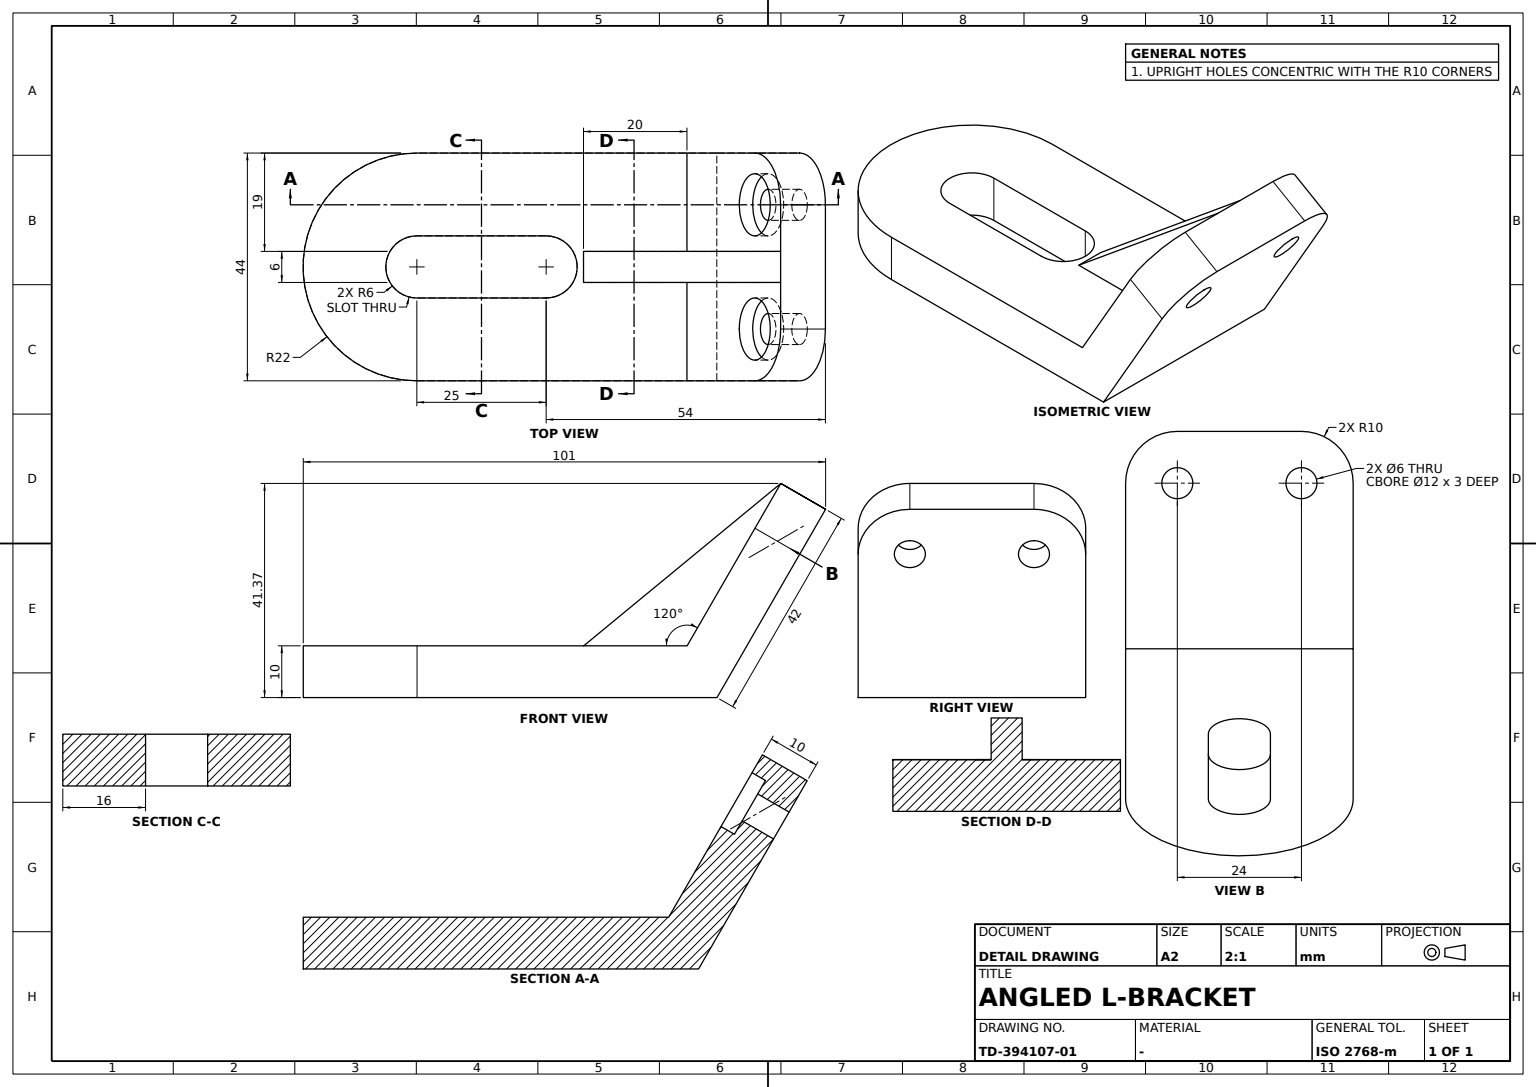
ISO-10303-21;
HEADER;
FILE_DESCRIPTION((''),'2;1');
FILE_NAME('','',(''),(''),'','','');
FILE_SCHEMA(('AUTOMOTIVE_DESIGN'));
ENDSEC;
DATA;
#1=APPLICATION_CONTEXT('');
#2=PRODUCT_CONTEXT('',#1,'mechanical');
#3=PRODUCT('','','',(#2));
#4=PRODUCT_DEFINITION_FORMATION('','',#3);
#5=PRODUCT_DEFINITION_CONTEXT('',#1,'design');
#6=PRODUCT_DEFINITION('','',#4,#5);
#7=PRODUCT_DEFINITION_SHAPE('','',#6);
#8=(LENGTH_UNIT()NAMED_UNIT(*)SI_UNIT(.MILLI.,.METRE.));
#9=(NAMED_UNIT(*)PLANE_ANGLE_UNIT()SI_UNIT($,.RADIAN.));
#10=(NAMED_UNIT(*)SI_UNIT($,.STERADIAN.)SOLID_ANGLE_UNIT());
#11=UNCERTAINTY_MEASURE_WITH_UNIT(LENGTH_MEASURE(0.005),#8,'distance_accuracy_value','');
#12=(GEOMETRIC_REPRESENTATION_CONTEXT(3)GLOBAL_UNCERTAINTY_ASSIGNED_CONTEXT((#11))GLOBAL_UNIT_ASSIGNED_CONTEXT((#8,#9,#10))REPRESENTATION_CONTEXT('',''));
#13=CARTESIAN_POINT('',(33.,6.,0.));
#14=VERTEX_POINT('',#13);
#15=CARTESIAN_POINT('',(33.,6.,10.));
#16=VERTEX_POINT('',#15);
#17=CARTESIAN_POINT('',(33.,6.,5.));
#18=DIRECTION('',(0.,0.,1.));
#19=VECTOR('',#18,1000.);
#20=LINE('',#17,#19);
#21=EDGE_CURVE('',#14,#16,#20,.T.);
#22=ORIENTED_EDGE('',*,*,#21,.T.);
#23=CARTESIAN_POINT('',(33.,-6.,10.));
#24=VERTEX_POINT('',#23);
#25=CARTESIAN_POINT('',(33.,0.,10.));
#26=DIRECTION('',(1.,0.,0.));
#27=AXIS2_PLACEMENT_3D('',#25,#18,#26);
#28=CIRCLE('',#27,6.);
#29=EDGE_CURVE('',#16,#24,#28,.T.);
#30=ORIENTED_EDGE('',*,*,#29,.T.);
#31=CARTESIAN_POINT('',(33.,-6.,0.));
#32=VERTEX_POINT('',#31);
#33=CARTESIAN_POINT('',(33.,-6.,5.));
#34=LINE('',#33,#19);
#35=EDGE_CURVE('',#32,#24,#34,.T.);
#36=ORIENTED_EDGE('',*,*,#35,.F.);
#37=CARTESIAN_POINT('',(33.,0.,0.));
#38=AXIS2_PLACEMENT_3D('',#37,#18,#26);
#39=CIRCLE('',#38,6.);
#40=EDGE_CURVE('',#14,#32,#39,.T.);
#41=ORIENTED_EDGE('',*,*,#40,.F.);
#42=EDGE_LOOP('',(#22,#30,#36,#41));
#43=FACE_BOUND('',#42,.T.);
#44=CARTESIAN_POINT('',(33.,0.,5.));
#45=AXIS2_PLACEMENT_3D('',#44,#18,#26);
#46=CYLINDRICAL_SURFACE('',#45,6.);
#47=ADVANCED_FACE('',(#43),#46,.F.);
#48=CARTESIAN_POINT('',(-4.339746,12.,27.51666));
#49=VERTEX_POINT('',#48);
#50=CARTESIAN_POINT('',(-7.339746,12.,32.712813));
#51=DIRECTION('',(0.866025404,0.,0.5));
#52=DIRECTION('',(0.5,0.,-0.866025404));
#53=AXIS2_PLACEMENT_3D('',#50,#51,#52);
#54=CIRCLE('',#53,6.);
#55=EDGE_CURVE('',#49,#49,#54,.T.);
#56=ORIENTED_EDGE('',*,*,#55,.F.);
#57=EDGE_LOOP('',(#56));
#58=FACE_BOUND('',#57,.T.);
#59=CARTESIAN_POINT('',(5.773503,3.,10.));
#60=VERTEX_POINT('',#59);
#61=CARTESIAN_POINT('',(5.773503,22.,10.));
#62=VERTEX_POINT('',#61);
#63=CARTESIAN_POINT('',(5.773503,0.,10.));
#64=DIRECTION('',(0.,1.,0.));
#65=VECTOR('',#64,1000.);
#66=LINE('',#63,#65);
#67=EDGE_CURVE('',#60,#62,#66,.T.);
#68=ORIENTED_EDGE('',*,*,#67,.T.);
#69=CARTESIAN_POINT('',(-7.339746,22.,32.712813));
#70=VERTEX_POINT('',#69);
#71=CARTESIAN_POINT('',(23.160254,22.,-20.114737));
#72=VECTOR('',#52,1000.);
#73=LINE('',#71,#72);
#74=EDGE_CURVE('',#70,#62,#73,.T.);
#75=ORIENTED_EDGE('',*,*,#74,.F.);
#76=CARTESIAN_POINT('',(-12.339746,12.,41.373067));
#77=VERTEX_POINT('',#76);
#78=CIRCLE('',#53,10.);
#79=EDGE_CURVE('',#70,#77,#78,.T.);
#80=ORIENTED_EDGE('',*,*,#79,.T.);
#81=CARTESIAN_POINT('',(-12.339746,3.,41.373067));
#82=VERTEX_POINT('',#81);
#83=CARTESIAN_POINT('',(-12.339746,-22.,41.373067));
#84=LINE('',#83,#65);
#85=EDGE_CURVE('',#82,#77,#84,.T.);
#86=ORIENTED_EDGE('',*,*,#85,.F.);
#87=CARTESIAN_POINT('',(8.660254,3.,5.));
#88=LINE('',#87,#72);
#89=EDGE_CURVE('',#82,#60,#88,.T.);
#90=ORIENTED_EDGE('',*,*,#89,.T.);
#91=EDGE_LOOP('',(#68,#75,#80,#86,#90));
#92=FACE_BOUND('',#91,.T.);
#93=AXIS2_PLACEMENT_3D('',#83,#51,#52);
#94=PLANE('',#93);
#95=ADVANCED_FACE('',(#58,#92),#94,.T.);
#96=CARTESIAN_POINT('',(58.,-6.,0.));
#97=VERTEX_POINT('',#96);
#98=CARTESIAN_POINT('',(58.,6.,0.));
#99=VERTEX_POINT('',#98);
#100=CARTESIAN_POINT('',(58.,0.,0.));
#101=AXIS2_PLACEMENT_3D('',#100,#18,#26);
#102=CIRCLE('',#101,6.);
#103=EDGE_CURVE('',#97,#99,#102,.T.);
#104=ORIENTED_EDGE('',*,*,#103,.F.);
#105=CARTESIAN_POINT('',(58.,-6.,10.));
#106=VERTEX_POINT('',#105);
#107=CARTESIAN_POINT('',(58.,-6.,5.));
#108=LINE('',#107,#19);
#109=EDGE_CURVE('',#97,#106,#108,.T.);
#110=ORIENTED_EDGE('',*,*,#109,.T.);
#111=CARTESIAN_POINT('',(58.,6.,10.));
#112=VERTEX_POINT('',#111);
#113=CARTESIAN_POINT('',(58.,0.,10.));
#114=AXIS2_PLACEMENT_3D('',#113,#18,#26);
#115=CIRCLE('',#114,6.);
#116=EDGE_CURVE('',#106,#112,#115,.T.);
#117=ORIENTED_EDGE('',*,*,#116,.T.);
#118=CARTESIAN_POINT('',(58.,6.,5.));
#119=LINE('',#118,#19);
#120=EDGE_CURVE('',#99,#112,#119,.T.);
#121=ORIENTED_EDGE('',*,*,#120,.F.);
#122=EDGE_LOOP('',(#104,#110,#117,#121));
#123=FACE_BOUND('',#122,.T.);
#124=CARTESIAN_POINT('',(58.,0.,5.));
#125=AXIS2_PLACEMENT_3D('',#124,#18,#26);
#126=CYLINDRICAL_SURFACE('',#125,6.);
#127=ADVANCED_FACE('',(#123),#126,.F.);
#128=CARTESIAN_POINT('',(-8.437822,-12.,28.614737));
#129=VERTEX_POINT('',#128);
#130=CARTESIAN_POINT('',(-9.937822,-12.,31.212813));
#131=AXIS2_PLACEMENT_3D('',#130,#51,#52);
#132=CIRCLE('',#131,3.);
#133=EDGE_CURVE('',#129,#129,#132,.T.);
#134=ORIENTED_EDGE('',*,*,#133,.F.);
#135=EDGE_LOOP('',(#134));
#136=FACE_BOUND('',#135,.T.);
#137=CARTESIAN_POINT('',(-6.937822,-12.,26.01666));
#138=VERTEX_POINT('',#137);
#139=CIRCLE('',#131,6.);
#140=EDGE_CURVE('',#138,#138,#139,.T.);
#141=ORIENTED_EDGE('',*,*,#140,.T.);
#142=EDGE_LOOP('',(#141));
#143=FACE_BOUND('',#142,.T.);
#144=CARTESIAN_POINT('',(6.062178,0.,3.5));
#145=AXIS2_PLACEMENT_3D('',#144,#51,#64);
#146=PLANE('',#145);
#147=ADVANCED_FACE('',(#136,#143),#146,.T.);
#148=CARTESIAN_POINT('',(-7.339746,-22.,32.712813));
#149=VERTEX_POINT('',#148);
#150=CARTESIAN_POINT('',(5.773503,-22.,10.));
#151=VERTEX_POINT('',#150);
#152=LINE('',#83,#72);
#153=EDGE_CURVE('',#149,#151,#152,.T.);
#154=ORIENTED_EDGE('',*,*,#153,.F.);
#155=CARTESIAN_POINT('',(-16.,-22.,27.712813));
#156=VERTEX_POINT('',#155);
#157=CARTESIAN_POINT('',(-7.403848,-22.,32.675804));
#158=VECTOR('',#51,1000.);
#159=LINE('',#157,#158);
#160=EDGE_CURVE('',#156,#149,#159,.T.);
#161=ORIENTED_EDGE('',*,*,#160,.F.);
#162=CARTESIAN_POINT('',(0.,-22.,0.));
#163=VERTEX_POINT('',#162);
#164=DIRECTION('',(-0.5,0.,0.866025404));
#165=VECTOR('',#164,1000.);
#166=LINE('',#162,#165);
#167=EDGE_CURVE('',#163,#156,#166,.T.);
#168=ORIENTED_EDGE('',*,*,#167,.F.);
#169=CARTESIAN_POINT('',(58.,-22.,0.));
#170=VERTEX_POINT('',#169);
#171=VECTOR('',#26,1000.);
#172=LINE('',#162,#171);
#173=EDGE_CURVE('',#163,#170,#172,.T.);
#174=ORIENTED_EDGE('',*,*,#173,.T.);
#175=CARTESIAN_POINT('',(58.,-22.,10.));
#176=VERTEX_POINT('',#175);
#177=CARTESIAN_POINT('',(58.,-22.,5.));
#178=LINE('',#177,#19);
#179=EDGE_CURVE('',#170,#176,#178,.T.);
#180=ORIENTED_EDGE('',*,*,#179,.T.);
#181=CARTESIAN_POINT('',(0.,-22.,10.));
#182=LINE('',#181,#171);
#183=EDGE_CURVE('',#151,#176,#182,.T.);
#184=ORIENTED_EDGE('',*,*,#183,.F.);
#185=EDGE_LOOP('',(#154,#161,#168,#174,#180,#184));
#186=FACE_BOUND('',#185,.T.);
#187=DIRECTION('',(0.,-1.,0.));
#188=AXIS2_PLACEMENT_3D('',#162,#187,#26);
#189=PLANE('',#188);
#190=ADVANCED_FACE('',(#186),#189,.T.);
#191=CARTESIAN_POINT('',(-12.339746,-12.,41.373067));
#192=VERTEX_POINT('',#191);
#193=CARTESIAN_POINT('',(-12.339746,-3.,41.373067));
#194=VERTEX_POINT('',#193);
#195=EDGE_CURVE('',#192,#194,#84,.T.);
#196=ORIENTED_EDGE('',*,*,#195,.F.);
#197=CARTESIAN_POINT('',(-7.339746,-12.,32.712813));
#198=AXIS2_PLACEMENT_3D('',#197,#51,#52);
#199=CIRCLE('',#198,10.);
#200=EDGE_CURVE('',#192,#149,#199,.T.);
#201=ORIENTED_EDGE('',*,*,#200,.T.);
#202=ORIENTED_EDGE('',*,*,#153,.T.);
#203=CARTESIAN_POINT('',(5.773503,-3.,10.));
#204=VERTEX_POINT('',#203);
#205=EDGE_CURVE('',#151,#204,#66,.T.);
#206=ORIENTED_EDGE('',*,*,#205,.T.);
#207=CARTESIAN_POINT('',(8.660254,-3.,5.));
#208=LINE('',#207,#72);
#209=EDGE_CURVE('',#194,#204,#208,.T.);
#210=ORIENTED_EDGE('',*,*,#209,.F.);
#211=EDGE_LOOP('',(#196,#201,#202,#206,#210));
#212=FACE_BOUND('',#211,.T.);
#213=CARTESIAN_POINT('',(-4.339746,-12.,27.51666));
#214=VERTEX_POINT('',#213);
#215=CIRCLE('',#198,6.);
#216=EDGE_CURVE('',#214,#214,#215,.T.);
#217=ORIENTED_EDGE('',*,*,#216,.F.);
#218=EDGE_LOOP('',(#217));
#219=FACE_BOUND('',#218,.T.);
#220=ADVANCED_FACE('',(#212,#219),#94,.T.);
#221=CARTESIAN_POINT('',(-17.5,12.,30.310889));
#222=VERTEX_POINT('',#221);
#223=CARTESIAN_POINT('',(-16.,12.,27.712813));
#224=DIRECTION('',(-0.866025404,0.,-0.5));
#225=AXIS2_PLACEMENT_3D('',#223,#224,#164);
#226=CIRCLE('',#225,3.);
#227=EDGE_CURVE('',#222,#222,#226,.T.);
#228=ORIENTED_EDGE('',*,*,#227,.F.);
#229=EDGE_LOOP('',(#228));
#230=FACE_BOUND('',#229,.T.);
#231=CARTESIAN_POINT('',(-17.5,-12.,30.310889));
#232=VERTEX_POINT('',#231);
#233=CARTESIAN_POINT('',(-16.,-12.,27.712813));
#234=AXIS2_PLACEMENT_3D('',#233,#224,#164);
#235=CIRCLE('',#234,3.);
#236=EDGE_CURVE('',#232,#232,#235,.T.);
#237=ORIENTED_EDGE('',*,*,#236,.F.);
#238=EDGE_LOOP('',(#237));
#239=FACE_BOUND('',#238,.T.);
#240=CARTESIAN_POINT('',(0.,22.,0.));
#241=VERTEX_POINT('',#240);
#242=CARTESIAN_POINT('',(0.,0.,0.));
#243=VECTOR('',#187,1000.);
#244=LINE('',#242,#243);
#245=EDGE_CURVE('',#241,#163,#244,.T.);
#246=ORIENTED_EDGE('',*,*,#245,.T.);
#247=ORIENTED_EDGE('',*,*,#167,.T.);
#248=CARTESIAN_POINT('',(-21.,-12.,36.373067));
#249=VERTEX_POINT('',#248);
#250=CIRCLE('',#234,10.);
#251=EDGE_CURVE('',#156,#249,#250,.T.);
#252=ORIENTED_EDGE('',*,*,#251,.T.);
#253=CARTESIAN_POINT('',(-21.,12.,36.373067));
#254=VERTEX_POINT('',#253);
#255=CARTESIAN_POINT('',(-21.,-22.,36.373067));
#256=LINE('',#255,#65);
#257=EDGE_CURVE('',#249,#254,#256,.T.);
#258=ORIENTED_EDGE('',*,*,#257,.T.);
#259=CARTESIAN_POINT('',(-16.,22.,27.712813));
#260=VERTEX_POINT('',#259);
#261=CIRCLE('',#225,10.);
#262=EDGE_CURVE('',#254,#260,#261,.T.);
#263=ORIENTED_EDGE('',*,*,#262,.T.);
#264=CARTESIAN_POINT('',(14.5,22.,-25.114737));
#265=LINE('',#264,#165);
#266=EDGE_CURVE('',#241,#260,#265,.T.);
#267=ORIENTED_EDGE('',*,*,#266,.F.);
#268=EDGE_LOOP('',(#246,#247,#252,#258,#263,#267));
#269=FACE_BOUND('',#268,.T.);
#270=AXIS2_PLACEMENT_3D('',#162,#224,#164);
#271=PLANE('',#270);
#272=ADVANCED_FACE('',(#230,#239,#269),#271,.T.);
#273=ORIENTED_EDGE('',*,*,#251,.F.);
#274=ORIENTED_EDGE('',*,*,#160,.T.);
#275=ORIENTED_EDGE('',*,*,#200,.F.);
#276=CARTESIAN_POINT('',(-12.403848,-12.,41.336058));
#277=LINE('',#276,#158);
#278=EDGE_CURVE('',#249,#192,#277,.T.);
#279=ORIENTED_EDGE('',*,*,#278,.F.);
#280=EDGE_LOOP('',(#273,#274,#275,#279));
#281=FACE_BOUND('',#280,.T.);
#282=CARTESIAN_POINT('',(-7.403848,-12.,32.675804));
#283=AXIS2_PLACEMENT_3D('',#282,#51,#164);
#284=CYLINDRICAL_SURFACE('',#283,10.);
#285=ADVANCED_FACE('',(#281),#284,.T.);
#286=ORIENTED_EDGE('',*,*,#29,.F.);
#287=CARTESIAN_POINT('',(0.,6.,10.));
#288=LINE('',#287,#171);
#289=EDGE_CURVE('',#16,#112,#288,.T.);
#290=ORIENTED_EDGE('',*,*,#289,.T.);
#291=ORIENTED_EDGE('',*,*,#116,.F.);
#292=CARTESIAN_POINT('',(0.,-6.,10.));
#293=LINE('',#292,#171);
#294=EDGE_CURVE('',#24,#106,#293,.T.);
#295=ORIENTED_EDGE('',*,*,#294,.F.);
#296=EDGE_LOOP('',(#286,#290,#291,#295));
#297=FACE_BOUND('',#296,.T.);
#298=CARTESIAN_POINT('',(58.,22.,10.));
#299=VERTEX_POINT('',#298);
#300=CARTESIAN_POINT('',(0.,22.,10.));
#301=DIRECTION('',(-1.,0.,0.));
#302=VECTOR('',#301,1000.);
#303=LINE('',#300,#302);
#304=EDGE_CURVE('',#299,#62,#303,.T.);
#305=ORIENTED_EDGE('',*,*,#304,.T.);
#306=ORIENTED_EDGE('',*,*,#67,.F.);
#307=CARTESIAN_POINT('',(25.773503,3.,10.));
#308=VERTEX_POINT('',#307);
#309=CARTESIAN_POINT('',(0.,3.,10.));
#310=LINE('',#309,#171);
#311=EDGE_CURVE('',#60,#308,#310,.T.);
#312=ORIENTED_EDGE('',*,*,#311,.T.);
#313=CARTESIAN_POINT('',(25.773503,-3.,10.));
#314=VERTEX_POINT('',#313);
#315=CARTESIAN_POINT('',(25.773503,0.,10.));
#316=LINE('',#315,#65);
#317=EDGE_CURVE('',#314,#308,#316,.T.);
#318=ORIENTED_EDGE('',*,*,#317,.F.);
#319=CARTESIAN_POINT('',(0.,-3.,10.));
#320=LINE('',#319,#171);
#321=EDGE_CURVE('',#204,#314,#320,.T.);
#322=ORIENTED_EDGE('',*,*,#321,.F.);
#323=ORIENTED_EDGE('',*,*,#205,.F.);
#324=ORIENTED_EDGE('',*,*,#183,.T.);
#325=CIRCLE('',#114,22.);
#326=EDGE_CURVE('',#176,#299,#325,.T.);
#327=ORIENTED_EDGE('',*,*,#326,.T.);
#328=EDGE_LOOP('',(#305,#306,#312,#318,#322,#323,#324,#327));
#329=FACE_BOUND('',#328,.T.);
#330=CARTESIAN_POINT('',(0.,0.,10.));
#331=AXIS2_PLACEMENT_3D('',#330,#18,#26);
#332=PLANE('',#331);
#333=ADVANCED_FACE('',(#297,#329),#332,.T.);
#334=ORIENTED_EDGE('',*,*,#278,.T.);
#335=ORIENTED_EDGE('',*,*,#195,.T.);
#336=LINE('',#83,#243);
#337=EDGE_CURVE('',#82,#194,#336,.T.);
#338=ORIENTED_EDGE('',*,*,#337,.F.);
#339=ORIENTED_EDGE('',*,*,#85,.T.);
#340=CARTESIAN_POINT('',(-12.403848,12.,41.336058));
#341=LINE('',#340,#158);
#342=EDGE_CURVE('',#254,#77,#341,.T.);
#343=ORIENTED_EDGE('',*,*,#342,.F.);
#344=ORIENTED_EDGE('',*,*,#257,.F.);
#345=EDGE_LOOP('',(#334,#335,#338,#339,#343,#344));
#346=FACE_BOUND('',#345,.T.);
#347=AXIS2_PLACEMENT_3D('',#255,#164,#51);
#348=PLANE('',#347);
#349=ADVANCED_FACE('',(#346),#348,.T.);
#350=CARTESIAN_POINT('',(-6.937822,12.,26.01666));
#351=VERTEX_POINT('',#350);
#352=CARTESIAN_POINT('',(-9.937822,12.,31.212813));
#353=AXIS2_PLACEMENT_3D('',#352,#51,#52);
#354=CIRCLE('',#353,6.);
#355=EDGE_CURVE('',#351,#351,#354,.T.);
#356=ORIENTED_EDGE('',*,*,#355,.T.);
#357=EDGE_LOOP('',(#356));
#358=FACE_BOUND('',#357,.T.);
#359=CARTESIAN_POINT('',(-8.437822,12.,28.614737));
#360=VERTEX_POINT('',#359);
#361=CIRCLE('',#353,3.);
#362=EDGE_CURVE('',#360,#360,#361,.T.);
#363=ORIENTED_EDGE('',*,*,#362,.F.);
#364=EDGE_LOOP('',(#363));
#365=FACE_BOUND('',#364,.T.);
#366=ADVANCED_FACE('',(#358,#365),#146,.T.);
#367=ORIENTED_EDGE('',*,*,#109,.F.);
#368=CARTESIAN_POINT('',(0.,-6.,0.));
#369=LINE('',#368,#171);
#370=EDGE_CURVE('',#32,#97,#369,.T.);
#371=ORIENTED_EDGE('',*,*,#370,.F.);
#372=ORIENTED_EDGE('',*,*,#35,.T.);
#373=ORIENTED_EDGE('',*,*,#294,.T.);
#374=EDGE_LOOP('',(#367,#371,#372,#373));
#375=FACE_BOUND('',#374,.T.);
#376=AXIS2_PLACEMENT_3D('',#31,#187,#26);
#377=PLANE('',#376);
#378=ADVANCED_FACE('',(#375),#377,.F.);
#379=ORIENTED_EDGE('',*,*,#209,.T.);
#380=ORIENTED_EDGE('',*,*,#321,.T.);
#381=DIRECTION('',(0.77207251,0.,-0.635534451));
#382=VECTOR('',#381,1000.);
#383=LINE('',#193,#382);
#384=EDGE_CURVE('',#194,#314,#383,.T.);
#385=ORIENTED_EDGE('',*,*,#384,.F.);
#386=EDGE_LOOP('',(#379,#380,#385));
#387=FACE_BOUND('',#386,.T.);
#388=CARTESIAN_POINT('',(0.,-3.,0.));
#389=AXIS2_PLACEMENT_3D('',#388,#64,#301);
#390=PLANE('',#389);
#391=ADVANCED_FACE('',(#387),#390,.F.);
#392=CARTESIAN_POINT('',(58.,22.,0.));
#393=VERTEX_POINT('',#392);
#394=CARTESIAN_POINT('',(58.,22.,5.));
#395=LINE('',#394,#19);
#396=EDGE_CURVE('',#393,#299,#395,.T.);
#397=ORIENTED_EDGE('',*,*,#396,.T.);
#398=ORIENTED_EDGE('',*,*,#326,.F.);
#399=ORIENTED_EDGE('',*,*,#179,.F.);
#400=CIRCLE('',#101,22.);
#401=EDGE_CURVE('',#170,#393,#400,.T.);
#402=ORIENTED_EDGE('',*,*,#401,.T.);
#403=EDGE_LOOP('',(#397,#398,#399,#402));
#404=FACE_BOUND('',#403,.T.);
#405=CYLINDRICAL_SURFACE('',#125,22.);
#406=ADVANCED_FACE('',(#404),#405,.T.);
#407=ORIENTED_EDGE('',*,*,#227,.T.);
#408=EDGE_LOOP('',(#407));
#409=FACE_BOUND('',#408,.T.);
#410=ORIENTED_EDGE('',*,*,#362,.T.);
#411=EDGE_LOOP('',(#410));
#412=FACE_BOUND('',#411,.T.);
#413=CARTESIAN_POINT('',(-23.716206,12.,23.257859));
#414=AXIS2_PLACEMENT_3D('',#413,#51,#64);
#415=CYLINDRICAL_SURFACE('',#414,3.);
#416=ADVANCED_FACE('',(#409,#412),#415,.F.);
#417=ORIENTED_EDGE('',*,*,#103,.T.);
#418=CARTESIAN_POINT('',(0.,6.,0.));
#419=LINE('',#418,#171);
#420=EDGE_CURVE('',#14,#99,#419,.T.);
#421=ORIENTED_EDGE('',*,*,#420,.F.);
#422=ORIENTED_EDGE('',*,*,#40,.T.);
#423=ORIENTED_EDGE('',*,*,#370,.T.);
#424=EDGE_LOOP('',(#417,#421,#422,#423));
#425=FACE_BOUND('',#424,.T.);
#426=ORIENTED_EDGE('',*,*,#401,.F.);
#427=ORIENTED_EDGE('',*,*,#173,.F.);
#428=ORIENTED_EDGE('',*,*,#245,.F.);
#429=LINE('',#240,#302);
#430=EDGE_CURVE('',#393,#241,#429,.T.);
#431=ORIENTED_EDGE('',*,*,#430,.F.);
#432=EDGE_LOOP('',(#426,#427,#428,#431));
#433=FACE_BOUND('',#432,.T.);
#434=AXIS2_PLACEMENT_3D('',#242,#18,#26);
#435=PLANE('',#434);
#436=ADVANCED_FACE('',(#425,#433),#435,.F.);
#437=ORIENTED_EDGE('',*,*,#236,.T.);
#438=EDGE_LOOP('',(#437));
#439=FACE_BOUND('',#438,.T.);
#440=ORIENTED_EDGE('',*,*,#133,.T.);
#441=EDGE_LOOP('',(#440));
#442=FACE_BOUND('',#441,.T.);
#443=CARTESIAN_POINT('',(-23.716206,-12.,23.257859));
#444=AXIS2_PLACEMENT_3D('',#443,#51,#64);
#445=CYLINDRICAL_SURFACE('',#444,3.);
#446=ADVANCED_FACE('',(#439,#442),#445,.F.);
#447=ORIENTED_EDGE('',*,*,#216,.T.);
#448=EDGE_LOOP('',(#447));
#449=FACE_BOUND('',#448,.T.);
#450=ORIENTED_EDGE('',*,*,#140,.F.);
#451=EDGE_LOOP('',(#450));
#452=FACE_BOUND('',#451,.T.);
#453=CARTESIAN_POINT('',(-8.638784,-12.,31.962813));
#454=AXIS2_PLACEMENT_3D('',#453,#51,#64);
#455=CYLINDRICAL_SURFACE('',#454,6.);
#456=ADVANCED_FACE('',(#449,#452),#455,.F.);
#457=ORIENTED_EDGE('',*,*,#337,.T.);
#458=ORIENTED_EDGE('',*,*,#384,.T.);
#459=ORIENTED_EDGE('',*,*,#317,.T.);
#460=LINE('',#81,#382);
#461=EDGE_CURVE('',#82,#308,#460,.T.);
#462=ORIENTED_EDGE('',*,*,#461,.F.);
#463=EDGE_LOOP('',(#457,#458,#459,#462));
#464=FACE_BOUND('',#463,.T.);
#465=CARTESIAN_POINT('',(-12.339746,0.,41.373067));
#466=DIRECTION('',(-0.635534451,0.,-0.77207251));
#467=DIRECTION('',(-0.77207251,0.,0.635534451));
#468=AXIS2_PLACEMENT_3D('',#465,#466,#467);
#469=PLANE('',#468);
#470=ADVANCED_FACE('',(#464),#469,.F.);
#471=ORIENTED_EDGE('',*,*,#430,.T.);
#472=ORIENTED_EDGE('',*,*,#266,.T.);
#473=CARTESIAN_POINT('',(-7.403848,22.,32.675804));
#474=LINE('',#473,#158);
#475=EDGE_CURVE('',#260,#70,#474,.T.);
#476=ORIENTED_EDGE('',*,*,#475,.T.);
#477=ORIENTED_EDGE('',*,*,#74,.T.);
#478=ORIENTED_EDGE('',*,*,#304,.F.);
#479=ORIENTED_EDGE('',*,*,#396,.F.);
#480=EDGE_LOOP('',(#471,#472,#476,#477,#478,#479));
#481=FACE_BOUND('',#480,.T.);
#482=AXIS2_PLACEMENT_3D('',#392,#64,#301);
#483=PLANE('',#482);
#484=ADVANCED_FACE('',(#481),#483,.T.);
#485=ORIENTED_EDGE('',*,*,#355,.F.);
#486=EDGE_LOOP('',(#485));
#487=FACE_BOUND('',#486,.T.);
#488=ORIENTED_EDGE('',*,*,#55,.T.);
#489=EDGE_LOOP('',(#488));
#490=FACE_BOUND('',#489,.T.);
#491=CARTESIAN_POINT('',(-8.638784,12.,31.962813));
#492=AXIS2_PLACEMENT_3D('',#491,#51,#64);
#493=CYLINDRICAL_SURFACE('',#492,6.);
#494=ADVANCED_FACE('',(#487,#490),#493,.F.);
#495=ORIENTED_EDGE('',*,*,#120,.T.);
#496=ORIENTED_EDGE('',*,*,#289,.F.);
#497=ORIENTED_EDGE('',*,*,#21,.F.);
#498=ORIENTED_EDGE('',*,*,#420,.T.);
#499=EDGE_LOOP('',(#495,#496,#497,#498));
#500=FACE_BOUND('',#499,.T.);
#501=AXIS2_PLACEMENT_3D('',#13,#187,#26);
#502=PLANE('',#501);
#503=ADVANCED_FACE('',(#500),#502,.T.);
#504=ORIENTED_EDGE('',*,*,#89,.F.);
#505=ORIENTED_EDGE('',*,*,#461,.T.);
#506=ORIENTED_EDGE('',*,*,#311,.F.);
#507=EDGE_LOOP('',(#504,#505,#506));
#508=FACE_BOUND('',#507,.T.);
#509=CARTESIAN_POINT('',(0.,3.,0.));
#510=AXIS2_PLACEMENT_3D('',#509,#64,#301);
#511=PLANE('',#510);
#512=ADVANCED_FACE('',(#508),#511,.T.);
#513=ORIENTED_EDGE('',*,*,#475,.F.);
#514=ORIENTED_EDGE('',*,*,#262,.F.);
#515=ORIENTED_EDGE('',*,*,#342,.T.);
#516=ORIENTED_EDGE('',*,*,#79,.F.);
#517=EDGE_LOOP('',(#513,#514,#515,#516));
#518=FACE_BOUND('',#517,.T.);
#519=CARTESIAN_POINT('',(-7.403848,12.,32.675804));
#520=AXIS2_PLACEMENT_3D('',#519,#51,#64);
#521=CYLINDRICAL_SURFACE('',#520,10.);
#522=ADVANCED_FACE('',(#518),#521,.T.);
#523=CLOSED_SHELL('',(#47,#95,#127,#147,#190,#220,#272,#285,#333,#349,#366,#378,#391,#406,#416,#436,#446,#456,#470,#484,#494,#503,#512,#522));
#524=MANIFOLD_SOLID_BREP('',#523);
#525=ADVANCED_BREP_SHAPE_REPRESENTATION('',(#524),#12);
#526=SHAPE_DEFINITION_REPRESENTATION(#7,#525);
ENDSEC;
END-ISO-10303-21;
